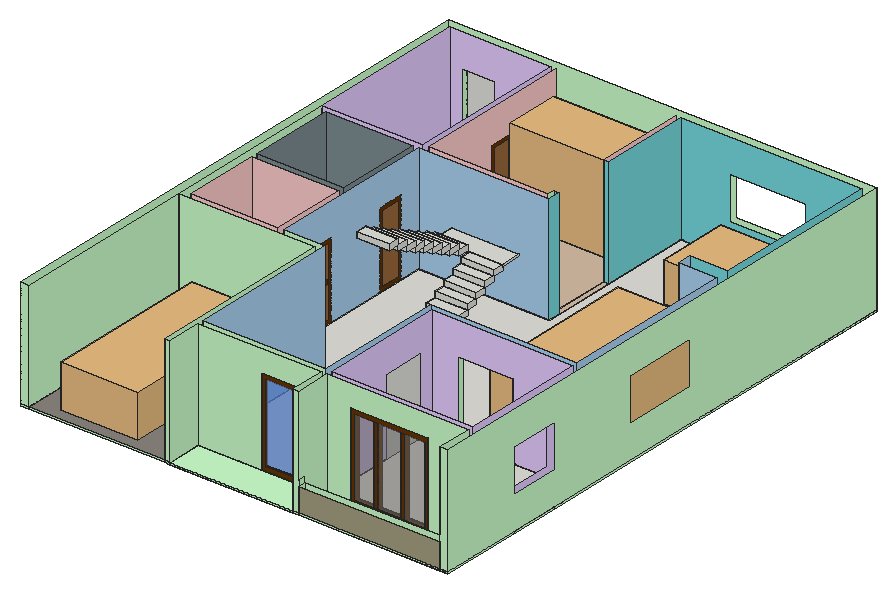
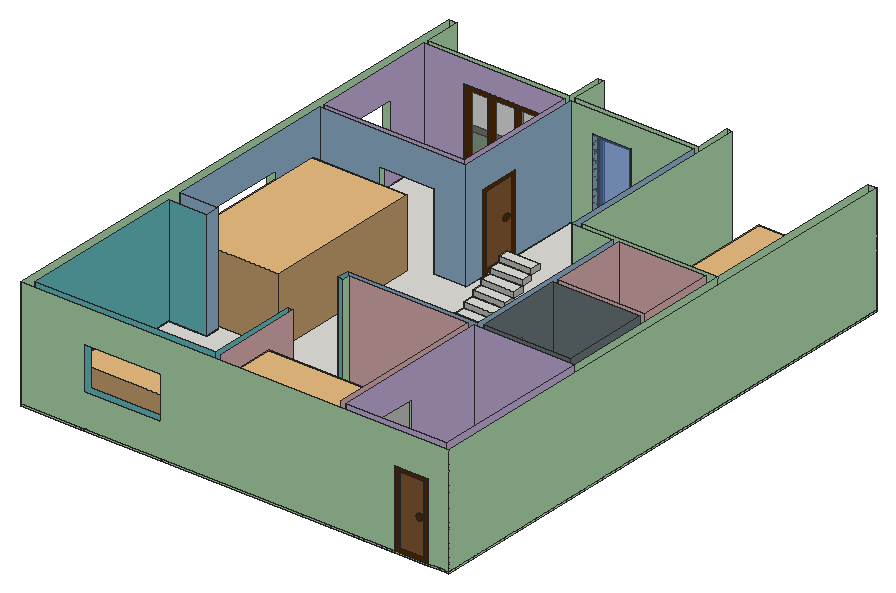
# SketchUp Ruby script. Lengths in inches.
U = 1.inch
M = Sketchup.active_model
def pt(a) = Geom::Point3d.new(a.map { |v| v * U })
def face(e, loops, mat)
  f = e.add_face(loops[0].map { |a| pt(a) })
  loops[1..].each { |l| e.add_face(l.map { |a| pt(a) }).erase! }
  f.material = f.back_material = mat if mat
  f
end
# faces: each face lists its corners as indices into pts; further lists are holes
def faces(e, pts, list, mat = nil) = list.each { |f| face(e, (f[0].is_a?(Array) ? f : [f]).map { |l| l.map { |i| pts[i] } }, mat) }
# xy, xz, yz: faces in a plane at the given z, y or x. An outline is a flat list of corners, or four numbers for a rectangle; further outlines are holes
def ring(l) = l.size == 4 ? [[l[0], l[1]], [l[2], l[1]], [l[2], l[3]], [l[0], l[3]]] : l.each_slice(2).to_a
def flat(e, list, mat, &to3) = list.each { |f| face(e, (f[0].is_a?(Array) ? f : [f]).map { |l| ring(l).map { |u, v| to3.(u, v) } }, mat) }
def xy(e, z, list, mat = nil) = flat(e, list, mat) { |x, y| [x, y, z] }
def xz(e, y, list, mat = nil) = flat(e, list, mat) { |x, z| [x, y, z] }
def yz(e, x, list, mat = nil) = flat(e, list, mat) { |y, z| [x, y, z] }
def lines(e, pts, list) = list.each { |a, b| e.add_line(pt(pts[a]), pt(pts[b])) }
# prism: a flat outline (further loops are holes) pulled along v
def prism(e, loops, v, mat = nil)
  f = face(e, loops, mat); d = Geom::Vector3d.new(v.map { |x| x * U })
  f.pushpull(f.normal.samedirection?(d) ? d.length : -d.length)
end
def box(e, o, s, mat = nil) = prism(e, [[o, [o[0] + s[0], o[1], o[2]], [o[0] + s[0], o[1] + s[1], o[2]], [o[0], o[1] + s[1], o[2]]]], [0, 0, s[2]], mat)
def at(x, y, z, deg = 0) = Geom::Transformation.translation(pt([x, y, z])) * Geom::Transformation.rotation(ORIGIN, Z_AXIS, deg.degrees)
def axes(o, x, y, z) = Geom::Transformation.new([*x, 0, *y, 0, *z, 0, *pt(o).to_a, 1])
def part(name) = M.definitions.add(name)
# library, detail: a bought-in or finely detailed component or shape, given as its bounding box
def library(name, o, s) = part(name).tap { |d| box(d.entities, o, s) }
def detail(e, o, s) = box(e.add_group.entities, o, s)
def put(e, d, t, mat = nil) = e.add_instance(d, t).tap { |i| i.material = mat if mat }
def group(e, t, mat = nil) = e.add_group.tap { |g| g.transformation = t; g.material = mat if mat }.entities
root = M.entities
M.materials.add("[Carrera Marble]").color = [207, 207, 207]
M.materials.add("[Color A01]").color = [255, 204, 204]
M.materials.add("[Color C08]").color = [102, 51, 0]
M.materials.add("[Color G01]").color = [204, 255, 204]
M.materials.add("[Color J01]").color = [229, 204, 255]
M.materials.add("[Concrete Pavers Block Multi]").color = [124, 140, 145]
M.materials.add("[Concrete Scored Jointless]").color = [140, 133, 127]
M.materials.add("[Formica Laminate Light]").color = [213, 189, 164]
M.materials.add("[Marble Carrara Gold Floor Tile]").color = [225, 223, 217]
M.materials.add("[Resin Blue]").color = [171, 210, 241]
M.materials.add("[Resin Turquoise]").color = [117, 218, 223]
M.materials.add("[Stone Coursed Rough]").color = [165, 160, 130]
M.materials.add("[Translucent Glass Blue]").color = [100, 149, 237]
M.materials["[Translucent Glass Blue]"].alpha = 0.5
M.materials.add("[Translucent Glass Gray]").color = [128, 128, 128]
M.materials["[Translucent Glass Gray]"].alpha = 0.5
M.materials.add("[Wood Floor]").color = [155, 105, 61]
c1 = part("Group\#8")
box(c1.entities,[0,0,0],[36,12,6])
c2 = part("Group\#10")
put(c2.entities,c1,at(0,24,12))
put(c2.entities,c1,at(0,96,48))
put(c2.entities,c1,at(0,36,18))
put(c2.entities,c1,at(0,48,24))
put(c2.entities,c1,at(0,72,36))
put(c2.entities,c1,at(0,84,42))
put(c2.entities,c1,at(0,0,0))
put(c2.entities,c1,at(0,12,6))
put(c2.entities,c1,at(0,60,30))
c3 = part("Group\#7")
xy(c3.entities,0,[[0,0,36,6]])
xy(c3.entities,4.09,[[4.09,0,31.91,2.0625]],"[Color C08]")
xy(c3.entities,79.91,[[4.09,0,31.91,2.0625]],"[Color C08]")
xy(c3.entities,84,[[0,0,36,6]],"[Color C08]")
xz(c3.entities,0,[[[0,0,36,84],[4.09,4.09,31.91,79.91]]],"[Color C08]")
xz(c3.entities,0.25,[[26.54,38.97,27.4,39.08,28.2,39.41,28.88,39.9375,29.41,40.625,29.74,41.42,29.85,42.28,29.74,43.14,29.41,43.9375,28.88,44.625,28.2,45.15,27.4,45.48,26.54,45.59,25.68,45.48,24.89,45.15,24.2,44.625,23.67,43.9375,23.34,43.14,23.23,42.28,23.34,41.42,23.67,40.625,24.2,39.9375,24.89,39.41,25.68,39.08]],"[Color C08]")
xz(c3.entities,2.0625,[[[4.09,4.09,31.91,79.91],[26.54,38.97,25.68,39.08,24.89,39.41,24.2,39.9375,23.67,40.625,23.34,41.42,23.23,42.28,23.34,43.14,23.67,43.9375,24.2,44.625,24.89,45.15,25.68,45.48,26.54,45.59,27.4,45.48,28.2,45.15,28.88,44.625,29.41,43.9375,29.74,43.14,29.85,42.28,29.74,41.42,29.41,40.625,28.88,39.9375,28.2,39.41,27.4,39.08]]],"[Wood Floor]")
xz(c3.entities,6,[[0,0,36,84]])
yz(c3.entities,0,[[0,0,6,84]],"[Color C08]")
yz(c3.entities,4.09,[[0,4.09,2.0625,79.91]],"[Color C08]")
yz(c3.entities,31.91,[[0,4.09,2.0625,79.91]],"[Color C08]")
yz(c3.entities,36,[[0,0,6,84]],"[Color C08]")
p = [[25.68,2.0625,39.08],[26.54,2.0625,38.97],[26.54,0.25,38.97],[25.68,0.25,39.08],[27.4,2.0625,39.08],[27.4,0.25,39.08],
  [24.89,2.0625,39.41],[24.89,0.25,39.41],[28.2,2.0625,39.41],[28.2,0.25,39.41],[24.2,2.0625,39.9375],[24.2,0.25,39.9375],
  [28.88,2.0625,39.9375],[28.88,0.25,39.9375],[23.67,2.0625,40.625],[23.67,0.25,40.625],[29.41,2.0625,40.625],[29.41,0.25,40.625],
  [23.34,2.0625,41.42],[23.34,0.25,41.42],[29.74,2.0625,41.42],[29.74,0.25,41.42],[23.23,2.0625,42.28],[23.23,0.25,42.28],
  [29.85,2.0625,42.28],[29.85,0.25,42.28],[23.34,2.0625,43.14],[23.34,0.25,43.14],[29.74,2.0625,43.14],[29.74,0.25,43.14],
  [23.67,2.0625,43.9375],[23.67,0.25,43.9375],[29.41,2.0625,43.9375],[29.41,0.25,43.9375],[24.2,2.0625,44.625],[24.2,0.25,44.625],
  [28.88,2.0625,44.625],[28.88,0.25,44.625],[24.89,2.0625,45.15],[24.89,0.25,45.15],[28.2,2.0625,45.15],[28.2,0.25,45.15],
  [25.68,2.0625,45.48],[25.68,0.25,45.48],[27.4,2.0625,45.48],[27.4,0.25,45.48],[26.54,2.0625,45.59],[26.54,0.25,45.59]]
faces(c3.entities,p,[[0,1,2,3],[1,4,5,2],[6,0,3,7],[4,8,9,5],[10,6,7,11],[8,12,13,9],[14,10,11,15],[12,16,17,13],
  [18,14,15,19],[16,20,21,17],[22,18,19,23],[20,24,25,21],[26,22,23,27],[24,28,29,25],[30,26,27,31],[28,32,33,29],
  [34,30,31,35],[32,36,37,33],[38,34,35,39],[36,40,41,37],[42,38,39,43],[40,44,45,41],[46,42,43,47],[44,46,47,45]],"[Color C08]")
c4 = library("Sofa set Collection\#1",[635.72,692.31,0],[158.93,122.75,75.39])
c5 = library("Dining Set",[0,0,0],[111.37,78.0625,43.36])
c6 = library("L-shaped kitchen",[55.71,-118.11,21.3],[196.85,118.11,96.45])
c7 = library("skp3430",[-10.67,-22.6875,-0.04],[21.34,45.28,11.76])
xy(root,-2,[[0,0,0,590,9.3125,590,9.3125,581,9,581,9,0],[159,0,159,207,9.3125,207,9.3125,405,120,405,120,490.74,126,490.74,126,405,258,405,258,412.4,264,412.4,264,399,120,399,120,375.1,114,375.1,114,399,18,399,18,303,114,303,114,345.1,120,345.1,120,278.47,114,278.47,114,297,18,297,18,213,114,213,114,248.47,120,248.47,120,213,165,213,165,45,234.6875,45,234.6875,39,165,39,165,0],[301,0,301,39,276.8125,39,276.8125,45,301,45,301,120.1875,307,120.1875,307,45,333.57,45,333.57,39,307,39,307,0],[307,0,463,9],[463,0,463,39,418.48,39,418.48,45,463,45,463,90.29,472,90.29,472,0],
  [[307,9,307,39,333.57,39,333.57,45,307,45,307,120.1875,301,120.1875,301,45,165,45,165,213,120,213,120,399,264,399,264,581,317.34,581,317.34,590,401.89,590,401.89,581,463,581,463,397.04,420.9375,397.04,420.9375,381.29,463,381.29,463,189,396.83,189,396.83,183,463,183,463,146.46,472,146.46,472,90.29,463,90.29,463,45,418.48,45,418.48,39,463,39,463,9],[301,168.1875,307,168.1875,307,183,336.83,183,336.83,189,301,189]],[234.6875,39,276.8125,45],[463,146.46,463,183,396.83,183,396.83,189,463,189,463,333.08,472,333.08,472,146.46],[301,168.1875,301,189,336.83,189,336.83,183,307,183,307,168.1875],[114,248.47,120,278.47],
  [463,333.08,463,381.29,420.9375,381.29,420.9375,397.04,463,397.04,463,581,401.89,581,401.89,590,472,590,472,333.08],[114,345.1,120,375.1],[258,412.4,264,481.74],[258,481.74,258,581,126,581,126,534.62,120,534.62,120,581,58.6875,581,58.6875,590,317.34,590,317.34,581,264,581,264,481.74],[9.3125,581,22.6875,590]],"[Color G01]")
xy(root,-2,[[9,0,159,207]],"[Concrete Scored Jointless]")
xy(root,-2,[[165,0,301,39],[18,213,114,297],[18,303,114,399],[9.3125,405,9.3125,581,22.6875,581,22.6875,590,58.6875,590,58.6875,581,120,581,120,534.62,126,534.62,126,581,258,581,258,405,126,405,126,490.74,120,490.74,120,405]],"[Marble Carrara Gold Floor Tile]")
xy(root,-0.25,[[[307,9,463,9,463,39,418.48,39,418.48,45,463,45,463,90.29,472,90.29,472,146.46,463,146.46,463,183,396.83,183,396.83,189,463,189,463,381.29,420.9375,381.29,420.9375,397.04,463,397.04,463,581,401.89,581,401.89,590,317.34,590,317.34,581,264,581,264,399,120,399,120,213,165,213,165,45,301,45,301,120.1875,307,120.1875,307,45,333.57,45,333.57,39,307,39],[301,168.1875,301,189,336.83,189,336.83,183,307,183,307,168.1875]]],"[Color G01]")
xy(root,0,[[18,213,114,297],[18,303,114,399]],"[Carrera Marble]")
xy(root,0,[[0,0,9,0,9,581,9.3125,581,9.3125,590,0,590],[159,0,165,0,165,39,234.6875,39,234.6875,45,165,45,165,213,120,213,120,248.47,114,248.47,114,213,18,213,18,297,114,297,114,278.47,120,278.47,120,345.1,114,345.1,114,303,18,303,18,399,114,399,114,375.1,120,375.1,120,399,264,399,264,412.4,258,412.4,258,405,126,405,126,490.74,120,490.74,120,405,9.3125,405,9.3125,207,159,207],[165,0,301,39],[301,0,307,0,307,39,333.57,39,333.57,45,307,45,307,120.1875,301,120.1875,301,45,276.8125,45,276.8125,39,301,39],[463,0,472,0,472,90.29,463,90.29,463,45,418.48,45,418.48,39,463,39],
  [234.6875,39,276.8125,45],[463,90.29,472,146.46],[463,146.46,472,146.46,472,333.08,463,333.08,463,189,396.83,189,396.83,183,463,183],[301,168.1875,307,168.1875,307,183,336.83,183,336.83,189,301,189],[9,207,9.3125,405],
  [114,248.47,120,278.47],[463,333.08,472,333.08,472,590,401.89,590,401.89,581,463,581,463,397.04,420.9375,397.04,420.9375,381.29,463,381.29],[114,345.1,120,375.1],[258,481.74,264,481.74,264,581,317.34,581,317.34,590,58.6875,590,58.6875,581,120,581,120,534.62,126,534.62,126,581,258,581],[9.3125,581,22.6875,590],
  [317.34,581,401.89,590]],"[Color G01]")
xy(root,0,[[9,0,9.3125,207],[9.3125,0,159,207]],"[Concrete Scored Jointless]")
xy(root,0,[[9.3125,405,120,405,120,490.74,126,490.74,126,405,258,405,258,581,126,581,126,534.62,120,534.62,120,581,58.6875,581,58.6875,590,22.6875,590,22.6875,581,9.3125,581],[258,412.4,264,481.74]],"[Formica Laminate Light]")
xy(root,0,[[[307,9,463,9,463,39,418.48,39,418.48,45,463,45,463,183,396.83,183,396.83,189,463,189,463,381.29,420.9375,381.29,420.9375,397.04,463,397.04,463,581,264,581,264,399,120,399,120,213,165,213,165,45,301,45,301,120.1875,307,120.1875,307,45,333.57,45,333.57,39,307,39],[301,168.1875,301,189,336.83,189,336.83,183,307,183,307,168.1875]],[9,405,9.3125,581]],"[Marble Carrara Gold Floor Tile]")
xz(root,0,[[0,-2,9,0],[9,-2,159,0],[159,-2,165,0],[165,-2,301,0],[301,-2,307,0],
  [307,-2,463,0],[463,-2,472,0],[0,0,9,120],[159,0,165,120],[301,0,307,120],
  [463,0,472,120]],"[Color G01]")
xz(root,0,[[307,0,463,25.9375]],"[Stone Coursed Rough]")
xz(root,9,[[307,-2,463,-0.25],[307,-0.25,463,0],[307,0,463,25.9375]],"[Color G01]")
xz(root,39,[[307,-2,333.57,-0.25],[418.48,-2,463,-0.25],[307,-0.25,333.57,0],[418.48,-0.25,463,0],[165,0,234.6875,0,234.6875,96,276.8125,96,276.8125,0,301,0,301,120,165,120],
  [307,0,333.57,0,333.57,96,418.48,96,418.48,0,463,0,463,120,307,120]],"[Color G01]")
xz(root,39,[[165,-2,234.6875,0],[234.6875,-2,276.8125,0],[276.8125,-2,301,0]],"[Marble Carrara Gold Floor Tile]")
xz(root,45,[[165,-2,185.25,-0.25],[185.25,-2,234.6875,-0.25],[234.6875,-2,271.8125,-0.25],[271.8125,-2,276.8125,-0.25],[276.8125,-2,301,-0.25],
  [307,-2,333.57,-0.25],[418.48,-2,463,-0.25],[165,-0.25,185.25,0],[185.25,-0.25,234.6875,0],[234.6875,-0.25,271.8125,0],
  [271.8125,-0.25,276.8125,0],[276.8125,-0.25,301,0],[307,-0.25,333.57,0],[418.48,-0.25,463,0],[165,0,165,120,301,120,301,0,276.8125,0,276.8125,96,234.6875,96,234.6875,0]],"[Color G01]")
xz(root,45,[[307,0,307,120,463,120,463,0,418.48,0,418.48,96,333.57,96,333.57,0]],"[Color J01]")
xz(root,90.29,[[463,-2,472,-0.25],[463,-0.25,472,0]],"[Color G01]")
xz(root,120.1875,[[301,-2,307,-0.25],[301,-0.25,307,0],[301,0,301,86.29,307,84,307,0]],"[Color G01]")
xz(root,146.46,[[463,-2,472,-0.25],[463,-0.25,472,0]],"[Color G01]")
xz(root,168.1875,[[301,-2,307,-0.25],[301,-0.25,307,0],[301,0,301,86.29,307,84,307,0]],"[Color G01]")
xz(root,183,[[307,-2,336.83,-0.25],[396.83,-2,463,-0.25],[307,-0.25,336.83,0],[396.83,-0.25,463,0]],"[Color G01]")
xz(root,183,[[307,0,336.83,0,336.83,84,396.83,84,396.83,0,463,0,463,120,307,120]],"[Color J01]")
xz(root,189,[[301,-2,336.83,-0.25],[396.83,-2,463,-0.25],[301,-0.25,336.83,0],[396.83,-0.25,463,0]],"[Color G01]")
xz(root,189,[[301,0,301,120,463,120,463,0,396.83,0,396.83,84,336.83,84,336.83,0]],"[Resin Blue]")
xz(root,207,[[9.3125,-2,159,0],[9,0,159,120]],"[Color G01]")
xz(root,207,[[9,-2,9.3125,0]],"[Concrete Scored Jointless]")
xz(root,213,[[18,0,114,120]],"[Color A01]")
xz(root,213,[[120,-2,165,-0.25],[120,-0.25,165,0],[120,0,165,120]],"[Color G01]")
xz(root,213,[[18,-2,114,0]],"[Marble Carrara Gold Floor Tile]")
xz(root,248.47,[[114,-2,120,0],[114,0,120,84]],"[Color G01]")
xz(root,278.47,[[114,-2,120,0],[114,0,120,84]],"[Color G01]")
xz(root,297,[[18,0,114,120]],"[Color A01]")
xz(root,297,[[18,-2,114,0]],"[Marble Carrara Gold Floor Tile]")
xz(root,303,[[18,0,114,120]],"[Concrete Pavers Block Multi]")
xz(root,303,[[18,-2,114,0]],"[Marble Carrara Gold Floor Tile]")
xz(root,333.08,[[463,-2,472,0]],"[Color G01]")
xz(root,345.1,[[114,-2,120,0],[114,0,120,84]],"[Color G01]")
xz(root,375.1,[[114,-2,120,0],[114,0,120,84]],"[Color G01]")
xz(root,381.29,[[420.9375,-2,463,-0.25],[420.9375,-0.25,463,0]],"[Color G01]")
xz(root,381.29,[[420.9375,0,463,120]],"[Resin Blue]")
xz(root,397.04,[[420.9375,-2,463,-0.25],[420.9375,-0.25,463,0]],"[Color G01]")
xz(root,397.04,[[420.9375,0,463,120]],"[Resin Turquoise]")
xz(root,399,[[120,-2,264,-0.25],[120,-0.25,264,0]],"[Color G01]")
xz(root,399,[[18,0,114,120]],"[Concrete Pavers Block Multi]")
xz(root,399,[[18,-2,114,0]],"[Marble Carrara Gold Floor Tile]")
xz(root,399,[[120,0,264,120]],"[Resin Blue]")
xz(root,405,[[126,0,258,120]],"[Color A01]")
xz(root,405,[[9,0,120,120]],"[Color J01]")
xz(root,405,[[9.3125,-2,120,0],[126,-2,258,0]],"[Marble Carrara Gold Floor Tile]")
xz(root,412.4,[[258,-2,264,0]],"[Color G01]")
xz(root,412.4,[[258,0,264,120]],"[Resin Turquoise]")
xz(root,481.74,[[258,-2,264,0]],"[Color G01]")
xz(root,481.74,[[258,0,264,120]],"[Resin Turquoise]")
xz(root,490.74,[[120,0,126,84]],"[Color G01]")
xz(root,490.74,[[120,-2,126,0]],"[Marble Carrara Gold Floor Tile]")
xz(root,534.62,[[120,0,126,28.25]],"[Color G01]")
xz(root,534.62,[[120,-2,126,0]],"[Marble Carrara Gold Floor Tile]")
xz(root,581,[[9,-2,9.3125,0],[264,-2,317.34,-0.25],[401.89,-2,463,-0.25],[264,-0.25,317.34,0],[401.89,-0.25,463,0],
  [126,0,258,28.25]],"[Color G01]")
xz(root,581,[[9,0,22.6875,0,22.6875,84,58.6875,84,58.6875,0,120,0,120,120,9,120]],"[Color J01]")
xz(root,581,[[9.3125,-2,22.6875,0],[58.6875,-2,120,0],[126,-2,258,0]],"[Marble Carrara Gold Floor Tile]")
xz(root,581,[[[264,0,463,120],[317.34,36,401.89,84]]],"[Resin Turquoise]")
xz(root,590,[[0,-2,9.3125,0],[9.3125,-2,22.6875,0],[22.6875,-2,58.6875,0],[58.6875,-2,317.34,0],[317.34,-2,401.89,-0.25],
  [401.89,-2,472,0],[317.34,-0.25,401.89,0],[[0,0,0,120,472,120,472,0,58.6875,0,58.6875,84,22.6875,84,22.6875,0],[317.34,36,401.89,84]]],"[Color G01]")
yz(root,0,[[0,-2,590,0],[0,0,590,120]],"[Color G01]")
yz(root,9,[[207,-2,405,0],[405,-2,581,0],[0,0,207,120],[207,0,405,120]],"[Color G01]")
yz(root,9,[[405,0,581,120]],"[Color J01]")
yz(root,9,[[0,-2,207,0]],"[Concrete Scored Jointless]")
yz(root,9.3125,[[207,-2,405,0],[581,-2,590,0]],"[Color G01]")
yz(root,9.3125,[[405,-2,581,0]],"[Marble Carrara Gold Floor Tile]")
yz(root,18,[[213,0,297,120]],"[Color A01]")
yz(root,18,[[303,0,399,120]],"[Concrete Pavers Block Multi]")
yz(root,18,[[213,-2,297,0],[303,-2,399,0]],"[Marble Carrara Gold Floor Tile]")
yz(root,22.6875,[[581,0,590,84]],"[Color G01]")
yz(root,22.6875,[[581,-2,590,0]],"[Marble Carrara Gold Floor Tile]")
yz(root,58.6875,[[581,0,590,28.25]],"[Color G01]")
yz(root,58.6875,[[581,-2,590,0]],"[Marble Carrara Gold Floor Tile]")
yz(root,114,[[213,0,213,120,297,120,297,0,278.47,0,278.47,84,248.47,84,248.47,0]],"[Color A01]")
yz(root,114,[[303,0,303,120,399,120,399,0,375.1,0,375.1,84,345.1,84,345.1,0]],"[Concrete Pavers Block Multi]")
yz(root,114,[[213,-2,248.47,0],[248.47,-2,278.47,0],[278.47,-2,297,0],[303,-2,345.1,0],[345.1,-2,375.1,0],
  [375.1,-2,399,0]],"[Marble Carrara Gold Floor Tile]")
yz(root,120,[[213,-2,248.47,-0.25],[248.47,-2,278.47,-0.25],[278.47,-2,345.1,-0.25],[345.1,-2,375.1,-0.25],[375.1,-2,399,-0.25],
  [213,-0.25,248.47,0],[248.47,-0.25,278.47,0],[278.47,-0.25,345.1,0],[345.1,-0.25,375.1,0],[375.1,-0.25,399,0]],"[Color G01]")
yz(root,120,[[405,0,405,120,581,120,581,0,534.62,0,534.62,84,490.74,84,490.74,0]],"[Color J01]")
yz(root,120,[[405,-2,490.74,0],[534.62,-2,581,0]],"[Marble Carrara Gold Floor Tile]")
yz(root,120,[[213,0,248.47,0,248.47,84,278.47,84,278.47,0,345.1,0,345.1,84,375.1,84,375.1,0,399,0,399,120,213,120]],"[Resin Blue]")
yz(root,126,[[405,0,490.74,0,490.74,84,534.62,84,534.62,28.25,581,28.25,581,120,405,120]],"[Color A01]")
yz(root,126,[[534.62,0,581,28.25]],"[Color G01]")
yz(root,126,[[405,-2,490.74,0],[534.62,-2,581,0]],"[Marble Carrara Gold Floor Tile]")
yz(root,159,[[0,0,207,120]],"[Color G01]")
yz(root,159,[[0,-2,207,0]],"[Concrete Scored Jointless]")
yz(root,165,[[45,-2,213,-0.25],[45,-0.25,213,0],[0,0,39,120]],"[Color G01]")
yz(root,165,[[0,-2,39,0]],"[Marble Carrara Gold Floor Tile]")
yz(root,165,[[45,0,213,120]],"[Resin Blue]")
yz(root,234.6875,[[39,-2,45,0],[39,0,45,96]],"[Color G01]")
yz(root,258,[[481.74,0,581,120]],"[Color A01]")
yz(root,258,[[405,0,412.4,120]],"[Color G01]")
yz(root,258,[[405,-2,412.4,0],[412.4,-2,481.74,0],[481.74,-2,581,0]],"[Marble Carrara Gold Floor Tile]")
yz(root,264,[[399,-2,412.4,-0.25],[412.4,-2,481.74,-0.25],[481.74,-2,581,-0.25],[399,-0.25,412.4,0],[412.4,-0.25,481.74,0],
  [481.74,-0.25,581,0]],"[Color G01]")
yz(root,264,[[399,0,412.4,120],[481.74,0,581,120]],"[Resin Turquoise]")
yz(root,276.8125,[[39,-2,45,0],[39,0,45,96]],"[Color G01]")
yz(root,301,[[45,-2,120.1875,-0.25],[168.1875,-2,189,-0.25],[45,-0.25,120.1875,0],[168.1875,-0.25,189,0],[0,0,39,120]],"[Color G01]")
yz(root,301,[[0,-2,39,0]],"[Marble Carrara Gold Floor Tile]")
yz(root,301,[[45,0,45,120,189,120,189,0,168.1875,0,168.1875,86.29,120.1875,86.29,120.1875,0]],"[Resin Blue]")
yz(root,307,[[0,-2,9,0],[9,-2,39,-0.25],[45,-2,120.1875,-0.25],[168.1875,-2,183,-0.25],[9,-0.25,39,0],
  [45,-0.25,120.1875,0],[168.1875,-0.25,183,0],[0,0,9,25.9375],[9,0,39,0,39,120,0,120,0,32.9375,9,32.9375]],"[Color G01]")
yz(root,307,[[45,0,120.1875,0,120.1875,84,168.1875,84,168.1875,0,183,0,183,120,45,120]],"[Color J01]")
yz(root,317.34,[[581,-2,590,-0.25],[581,-0.25,590,0]],"[Color G01]")
yz(root,333.57,[[39,-2,45,-0.25],[39,-0.25,45,0],[39,0,45,96]],"[Color G01]")
yz(root,336.83,[[183,-2,189,-0.25],[183,-0.25,189,0],[183,0,189,84]],"[Color G01]")
yz(root,396.83,[[183,-2,189,-0.25],[183,-0.25,189,0],[183,0,189,84]],"[Color G01]")
yz(root,401.89,[[581,-2,590,-0.25],[581,-0.25,590,0]],"[Color G01]")
yz(root,418.48,[[39,-2,45,-0.25],[39,-0.25,45,0],[39,0,45,96]],"[Color G01]")
yz(root,420.9375,[[381.29,-2,397.04,-0.25],[381.29,-0.25,397.04,0]],"[Color G01]")
yz(root,420.9375,[[381.29,0,397.04,120]],"[Resin Blue]")
yz(root,463,[[0,-2,9,0],[9,-2,39,-0.25],[45,-2,90.29,-0.25],[146.46,-2,183,-0.25],[189,-2,333.08,-0.25],
  [333.08,-2,381.29,-0.25],[397.04,-2,581,-0.25],[9,-0.25,39,0],[45,-0.25,90.29,0],[146.46,-0.25,183,0],
  [189,-0.25,333.08,0],[333.08,-0.25,381.29,0],[397.04,-0.25,581,0],[0,0,9,25.9375],[9,0,9,32.9375,0,32.9375,0,120,39,120,39,0]],"[Color G01]")
yz(root,463,[[[45,0,183,120],[90.29,36,146.46,84]]],"[Color J01]")
yz(root,463,[[[189,0,381.29,120],[249.52,36,333.08,84]]],"[Resin Blue]")
yz(root,463,[[397.04,0,581,120]],"[Resin Turquoise]")
yz(root,472,[[0,-2,90.29,0],[90.29,-2,146.46,-0.25],[146.46,-2,333.08,0],[333.08,-2,590,0],[90.29,-0.25,146.46,0],
  [[0,0,590,120],[249.52,36,333.08,84],[90.29,36,146.46,84]]],"[Color G01]")
g1 = group(root,at(156.39,267.6875,-0.25))
box(g1,[0,108,52.0625],[74.6875,23.3125,1.9375])
put(g1,c2,at(38.6875,0,0))
put(g1,c2,at(36.4375,108,54,-180))
g2 = group(root,at(333.09,39,0))
xy(g2,0,[[0,0,85.39,5.875]])
xy(g2,4.92,[[4.05,0,26.02,0.75],[26.02,0,30.01,5.875],[30.01,0,55.24,0.75],[55.24,0,59.23,5.875],[59.23,0,81.34,0.75],
  [4.05,0.75,26.02,5.875],[30.01,0.75,55.24,5.875],[59.23,0.75,81.34,5.875]],"[Color C08]")
xy(g2,91.08,[[4.05,0,26.02,0.75],[26.02,0,30.01,5.875],[30.01,0,55.24,0.75],[55.24,0,59.23,5.875],[59.23,0,81.34,0.75],
  [4.05,0.75,26.02,5.875],[30.01,0.75,55.24,5.875],[59.23,0.75,81.34,5.875]])
xy(g2,96,[[0,0,85.39,5.875]],"[Color C08]")
xz(g2,0,[[[0,0,85.39,96],[4.05,4.92,81.34,91.08]],[26.02,4.92,30.01,91.08],[55.24,4.92,59.23,91.08]],"[Color C08]")
xz(g2,0.75,[[4.05,4.92,26.02,91.08],[30.01,4.92,55.24,91.08],[59.23,4.92,81.34,91.08]],"[Translucent Glass Gray]")
xz(g2,5.875,[[[0,0,85.39,96],[4.05,4.92,81.34,91.08]],[26.02,4.92,30.01,91.08],[55.24,4.92,59.23,91.08]],"[Color C08]")
yz(g2,0,[[0,0,5.875,96]],"[Color C08]")
yz(g2,4.05,[[0,4.92,0.75,91.08],[0.75,4.92,5.875,91.08]],"[Color C08]")
yz(g2,26.02,[[0,4.92,0.75,91.08]])
yz(g2,26.02,[[0.75,4.92,5.875,91.08]],"[Color C08]")
yz(g2,30.01,[[0,4.92,0.75,91.08],[0.75,4.92,5.875,91.08]],"[Color C08]")
yz(g2,55.24,[[0,4.92,0.75,91.08],[0.75,4.92,5.875,91.08]],"[Color C08]")
yz(g2,59.23,[[0,4.92,0.75,91.08],[0.75,4.92,5.875,91.08]],"[Color C08]")
yz(g2,81.34,[[0,4.92,0.75,91.08],[0.75,4.92,5.875,91.08]],"[Color C08]")
yz(g2,85.39,[[0,0,5.875,96]],"[Color C08]")
put(root,c3,axes([120,345.16,0],[0,0.83333,0],[-0.56,0,0],[0,0,1]))
put(root,c3,axes([120,248.47,0],[0,0.83333,0],[-0.56,0,0],[0,0,1]))
put(root,c4,axes([-237.95,1084.5,0],[0,-1.1131,0],[0.86,0,0],[0,0,1]))
put(root,c5,at(322.6875,484.04,0))
put(root,c3,axes([301,168.1875,0],[0,-1.33333,0],[1,0,0],[0,0,1.02728]))
put(root,c3,axes([126,490.74,0],[0,1.21875,0],[-0.56,0,0],[0,0,1]))
put(root,c3,axes([58.6875,590,0],[-1,0,0],[0,-0.56,0],[0,0,1]))
put(root,c6,axes([88.64,576.42,-21.03],[0.67056,0,0],[0,0.51559,0],[0,0,0.98757]))
put(root,c7,axes([76.36,103.91,0.17],[4,0,0],[0,4,0],[0,0,4]))
g3 = group(root,at(234.6875,39,0.24))
xy(g3,0,[[0,0,42.125,6]])
xy(g3,4.66,[[4.79,0,37.34,2.0625]],"[Color C08]")
xy(g3,91.1,[[4.79,0,37.34,2.0625]],"[Color C08]")
xy(g3,95.76,[[0,0,42.125,6]],"[Color C08]")
xz(g3,0,[[[0,0,42.125,95.76],[4.79,4.66,37.34,91.1]]],"[Color C08]")
xz(g3,2.0625,[[4.79,4.66,37.34,91.1]],"[Translucent Glass Blue]")
xz(g3,6,[[0,0,42.125,95.76]],"[Translucent Glass Blue]")
yz(g3,0,[[0,0,6,95.76]],"[Color C08]")
yz(g3,4.79,[[0,4.66,2.0625,91.1]],"[Color C08]")
yz(g3,37.34,[[0,4.66,2.0625,91.1]],"[Color C08]")
yz(g3,42.125,[[0,0,6,95.76]],"[Color C08]")
